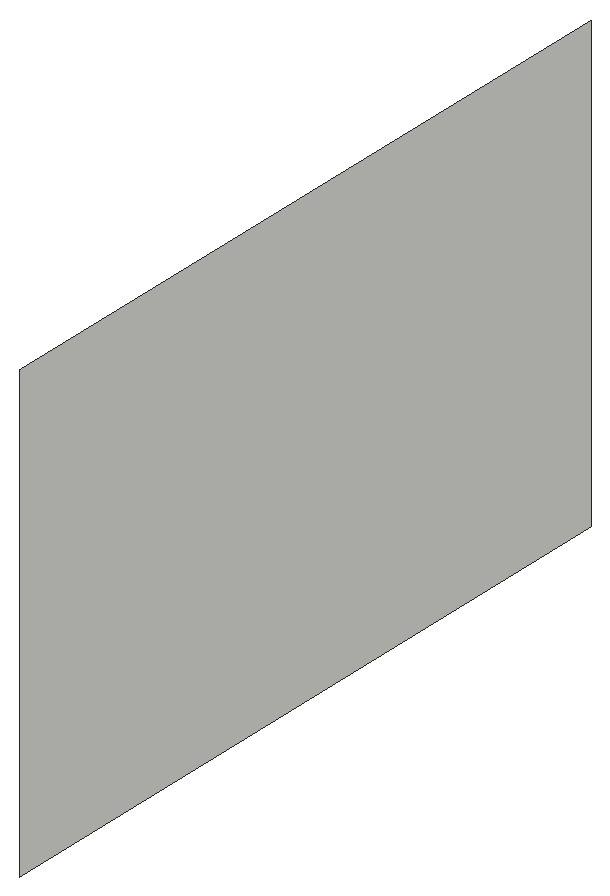
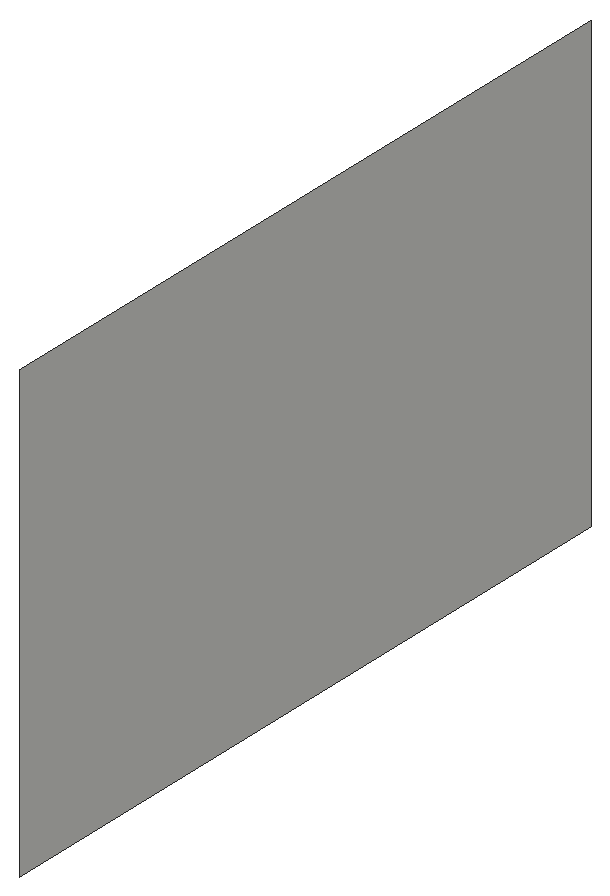
# SketchUp Ruby script. Lengths in inches.
U = 1.inch
M = Sketchup.active_model
def pt(a) = Geom::Point3d.new(a.map { |v| v * U })
def face(e, loops, mat)
  f = e.add_face(loops[0].map { |a| pt(a) })
  loops[1..].each { |l| e.add_face(l.map { |a| pt(a) }).erase! }
  f.material = f.back_material = mat if mat
  f
end
# faces: each face lists its corners as indices into pts; further lists are holes
def faces(e, pts, list, mat = nil) = list.each { |f| face(e, (f[0].is_a?(Array) ? f : [f]).map { |l| l.map { |i| pts[i] } }, mat) }
# xy, xz, yz: faces in a plane at the given z, y or x. An outline is a flat list of corners, or four numbers for a rectangle; further outlines are holes
def ring(l) = l.size == 4 ? [[l[0], l[1]], [l[2], l[1]], [l[2], l[3]], [l[0], l[3]]] : l.each_slice(2).to_a
def flat(e, list, mat, &to3) = list.each { |f| face(e, (f[0].is_a?(Array) ? f : [f]).map { |l| ring(l).map { |u, v| to3.(u, v) } }, mat) }
def xy(e, z, list, mat = nil) = flat(e, list, mat) { |x, y| [x, y, z] }
def xz(e, y, list, mat = nil) = flat(e, list, mat) { |x, z| [x, y, z] }
def yz(e, x, list, mat = nil) = flat(e, list, mat) { |y, z| [x, y, z] }
def lines(e, pts, list) = list.each { |a, b| e.add_line(pt(pts[a]), pt(pts[b])) }
# prism: a flat outline (further loops are holes) pulled along v
def prism(e, loops, v, mat = nil)
  f = face(e, loops, mat); d = Geom::Vector3d.new(v.map { |x| x * U })
  f.pushpull(f.normal.samedirection?(d) ? d.length : -d.length)
end
def box(e, o, s, mat = nil) = prism(e, [[o, [o[0] + s[0], o[1], o[2]], [o[0] + s[0], o[1] + s[1], o[2]], [o[0], o[1] + s[1], o[2]]]], [0, 0, s[2]], mat)
def at(x, y, z, deg = 0) = Geom::Transformation.translation(pt([x, y, z])) * Geom::Transformation.rotation(ORIGIN, Z_AXIS, deg.degrees)
def axes(o, x, y, z) = Geom::Transformation.new([*x, 0, *y, 0, *z, 0, *pt(o).to_a, 1])
def part(name) = M.definitions.add(name)
# library, detail: a bought-in or finely detailed component or shape, given as its bounding box
def library(name, o, s) = part(name).tap { |d| box(d.entities, o, s) }
def detail(e, o, s) = box(e.add_group.entities, o, s)
def put(e, d, t, mat = nil) = e.add_instance(d, t).tap { |i| i.material = mat if mat }
def group(e, t, mat = nil) = e.add_group.tap { |g| g.transformation = t; g.material = mat if mat }.entities
root = M.entities
yz(root,211.5,[[364.57,103.6875,374.19,109.8125]])
